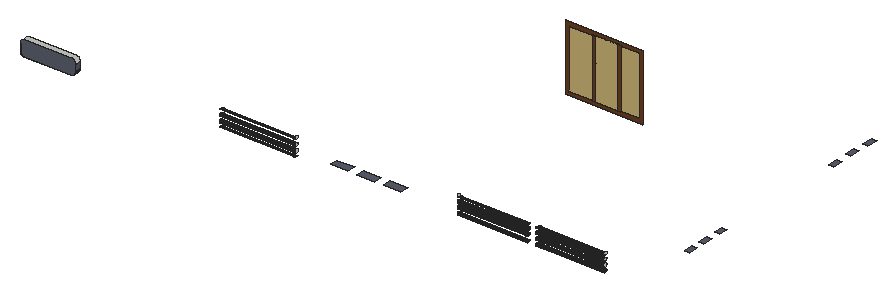
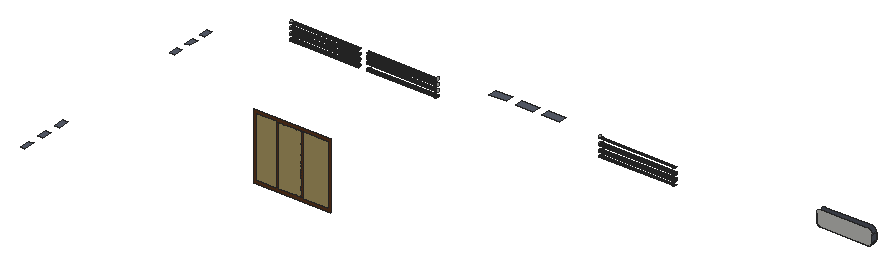
# SketchUp Ruby script. Lengths in inches.
U = 1.inch
M = Sketchup.active_model
def pt(a) = Geom::Point3d.new(a.map { |v| v * U })
def face(e, loops, mat)
  f = e.add_face(loops[0].map { |a| pt(a) })
  loops[1..].each { |l| e.add_face(l.map { |a| pt(a) }).erase! }
  f.material = f.back_material = mat if mat
  f
end
# faces: each face lists its corners as indices into pts; further lists are holes
def faces(e, pts, list, mat = nil) = list.each { |f| face(e, (f[0].is_a?(Array) ? f : [f]).map { |l| l.map { |i| pts[i] } }, mat) }
# xy, xz, yz: faces in a plane at the given z, y or x. An outline is a flat list of corners, or four numbers for a rectangle; further outlines are holes
def ring(l) = l.size == 4 ? [[l[0], l[1]], [l[2], l[1]], [l[2], l[3]], [l[0], l[3]]] : l.each_slice(2).to_a
def flat(e, list, mat, &to3) = list.each { |f| face(e, (f[0].is_a?(Array) ? f : [f]).map { |l| ring(l).map { |u, v| to3.(u, v) } }, mat) }
def xy(e, z, list, mat = nil) = flat(e, list, mat) { |x, y| [x, y, z] }
def xz(e, y, list, mat = nil) = flat(e, list, mat) { |x, z| [x, y, z] }
def yz(e, x, list, mat = nil) = flat(e, list, mat) { |y, z| [x, y, z] }
def lines(e, pts, list) = list.each { |a, b| e.add_line(pt(pts[a]), pt(pts[b])) }
# prism: a flat outline (further loops are holes) pulled along v
def prism(e, loops, v, mat = nil)
  f = face(e, loops, mat); d = Geom::Vector3d.new(v.map { |x| x * U })
  f.pushpull(f.normal.samedirection?(d) ? d.length : -d.length)
end
def box(e, o, s, mat = nil) = prism(e, [[o, [o[0] + s[0], o[1], o[2]], [o[0] + s[0], o[1] + s[1], o[2]], [o[0], o[1] + s[1], o[2]]]], [0, 0, s[2]], mat)
def at(x, y, z, deg = 0) = Geom::Transformation.translation(pt([x, y, z])) * Geom::Transformation.rotation(ORIGIN, Z_AXIS, deg.degrees)
def axes(o, x, y, z) = Geom::Transformation.new([*x, 0, *y, 0, *z, 0, *pt(o).to_a, 1])
def part(name) = M.definitions.add(name)
# library, detail: a bought-in or finely detailed component or shape, given as its bounding box
def library(name, o, s) = part(name).tap { |d| box(d.entities, o, s) }
def detail(e, o, s) = box(e.add_group.entities, o, s)
def put(e, d, t, mat = nil) = e.add_instance(d, t).tap { |i| i.material = mat if mat }
def group(e, t, mat = nil) = e.add_group.tap { |g| g.transformation = t; g.material = mat if mat }.entities
root = M.entities
M.materials.add("[Color M07]").color = [58, 58, 58]
M.materials.add("[Formica Laminate Dark]").color = [89, 94, 107]
M.materials.add("[Window Covering 02]").color = [199, 178, 115]
M.materials.add("[Wood Veneer 01]").color = [107, 62, 33]
xy(root,135.12,[[23.08,274.68,149.38,289.93]],"[Formica Laminate Dark]")
xy(root,149.91,[[1639.03,943.34,1652.28,971.59],[1639.03,1000.59,1652.28,1028.84],[1639.03,1058.41,1652.28,1086.66]],"[Formica Laminate Dark]")
xy(root,155.0625,[[1639.03,462.79,1652.28,487.66],[1639.03,510.85,1652.28,535.72],[1639.03,562.72,1652.28,587.6]],"[Formica Laminate Dark]")
xy(root,155.26,[[832.8125,288.14,879.5,309.57],[902.5,288.14,949.1875,309.57],[974.4375,288.14,1021.125,309.57]],"[Formica Laminate Dark]")
xz(root,274.68,[[23.08,135.12,149.38,135.12,150.95,135.23,152.5,135.53,153.99,136.04,155.4,136.74,156.71,137.61,157.9,138.65,158.9375,139.84,159.8125,141.15,160.51,142.56,161.02,144.05,161.32,145.6,161.43,147.17,161.43,162.99,161.32,164.68,160.99,166.34,160.44,167.94,159.69,169.46,158.75,170.87,157.64,172.14,156.36,173.26,154.96,174.2,153.4375,174.95,151.83,175.49,150.17,175.82,148.48,175.94,26.4,175.94,24.71,175.82,23.04,175.49,21.4375,174.95,19.91,174.2,18.5,173.25,17.23,172.14,16.11,170.86,15.17,169.45,14.42,167.93,13.87,166.32,13.54,164.66,13.43,162.96,13.43,144.77,13.51,143.51,13.76,142.27,14.16,141.08,14.72,139.95,15.42,138.9,16.25,137.95,17.2,137.12,18.25,136.42,19.38,135.86,20.58,135.45,21.82,135.21]],"[Formica Laminate Dark]")
xz(root,289.93,[[23.08,135.12,21.82,135.21,20.58,135.45,19.38,135.86,18.25,136.42,17.2,137.12,16.25,137.95,15.42,138.9,14.72,139.95,14.16,141.08,13.76,142.27,13.51,143.51,13.43,144.77,13.43,162.96,13.54,164.66,13.87,166.32,14.42,167.93,15.17,169.45,16.11,170.86,17.23,172.14,18.5,173.25,19.91,174.2,21.4375,174.95,23.04,175.49,24.71,175.82,26.4,175.94,148.48,175.94,150.17,175.82,151.83,175.49,153.4375,174.95,154.96,174.2,156.36,173.26,157.64,172.14,158.75,170.87,159.69,169.46,160.44,167.94,160.99,166.34,161.32,164.68,161.43,162.99,161.43,147.17,161.32,145.6,161.02,144.05,160.51,142.56,159.8125,141.15,158.9375,139.84,157.9,138.65,156.71,137.61,155.4,136.74,153.99,136.04,152.5,135.53,150.95,135.23,149.38,135.12]])
xz(root,868.79,[[1005.76,135.02,1068.89,293.73],[1077.3,135.02,1134.57,293.73],[1142.99,135.02,1193.04,293.73]],"[Window Covering 02]")
xz(root,868.79,[[[996.55,125.8125,1202.24,302.9375],[1005.76,135.02,1193.04,293.73]],[1068.89,135.02,1077.3,293.73],[1134.57,135.02,1142.99,293.73]],"[Wood Veneer 01]")
yz(root,13.43,[[274.68,144.77,289.93,162.96]],"[Formica Laminate Dark]")
yz(root,161.43,[[274.68,147.17,289.93,162.99]],"[Formica Laminate Dark]")
yz(root,716.4,[[319.3,129.24,320.31,129.37,321.24,129.76,322.04,130.375,322.66,131.18,323.05,132.11,323.18,133.11,323.05,134.12,322.66,135.05,322.04,135.85,321.24,136.47,320.31,136.86,319.3,136.99,318.3,136.86,317.37,136.47,316.56,135.85,315.95,135.05,315.5625,134.12,315.43,133.11,315.5625,132.11,315.95,131.18,316.56,130.375,317.37,129.76,318.3,129.37],[319.3,144.8,320.31,144.93,321.24,145.32,322.04,145.9375,322.66,146.74,323.05,147.67,323.18,148.68,323.05,149.68,322.66,150.61,322.04,151.42,321.24,152.03,320.31,152.42,319.3,152.55,318.3,152.42,317.37,152.03,316.56,151.42,315.95,150.61,315.5625,149.68,315.43,148.68,315.5625,147.67,315.95,146.74,316.56,145.9375,317.37,145.32,318.3,144.93],[319.3,161.86,320.31,162,321.24,162.38,322.04,163,322.66,163.8,323.05,164.74,323.18,165.74,323.05,166.74,322.66,167.68,322.04,168.48,321.24,169.09,320.31,169.48,319.3,169.61,318.3,169.48,317.37,169.09,316.56,168.48,315.95,167.68,315.5625,166.74,315.43,165.74,315.5625,164.74,315.95,163.8,316.56,163,317.37,162.38,318.3,162]])
yz(root,1134.85,[[337.34,134.02,336.35,134.15,335.43,134.53,334.65,135.13,334.04,135.92,333.66,136.84,333.53,137.83,333.66,138.82,334.04,139.74,334.65,140.53,335.43,141.13,336.35,141.51,337.34,141.64,338.33,141.51,339.25,141.13,340.04,140.53,340.64,139.74,341.02,138.82,341.15,137.83,341.02,136.84,340.64,135.92,340.04,135.13,339.25,134.53,338.33,134.15],[337.34,147.52,336.35,147.65,335.43,148.03,334.65,148.63,334.04,149.42,333.66,150.34,333.53,151.33,333.66,152.32,334.04,153.24,334.65,154.03,335.43,154.63,336.35,155.01,337.34,155.14,338.33,155.01,339.25,154.63,340.04,154.03,340.64,153.24,341.02,152.32,341.15,151.33,341.02,150.34,340.64,149.42,340.04,148.63,339.25,148.03,338.33,147.65],[337.34,161.02,336.35,161.15,335.43,161.53,334.65,162.13,334.04,162.92,333.66,163.84,333.53,164.83,333.66,165.82,334.04,166.74,334.65,167.53,335.43,168.13,336.35,168.51,337.34,168.64,338.33,168.51,339.25,168.13,340.04,167.53,340.64,166.74,341.02,165.82,341.15,164.83,341.02,163.84,340.64,162.92,340.04,162.13,339.25,161.53,338.33,161.15]])
yz(root,1527,[[337.76,132.85,338.75,132.98,339.67,133.36,340.46,133.97,341.0625,134.76,341.44,135.67,341.57,136.66,341.44,137.65,341.0625,138.57,340.46,139.36,339.67,139.96,338.75,140.34,337.76,140.47,336.77,140.34,335.85,139.96,335.06,139.36,334.46,138.57,334.08,137.65,333.95,136.66,334.08,135.67,334.46,134.76,335.06,133.97,335.85,133.36,336.77,132.98],[337.76,146.47,338.75,146.6,339.67,146.98,340.46,147.59,341.0625,148.38,341.44,149.3,341.57,150.29,341.44,151.27,341.0625,152.19,340.46,152.98,339.67,153.59,338.75,153.97,337.76,154.1,336.77,153.97,335.85,153.59,335.06,152.98,334.46,152.19,334.08,151.27,333.95,150.29,334.08,149.3,334.46,148.38,335.06,147.59,335.85,146.98,336.77,146.6],[337.76,160.47,338.75,160.6,339.67,160.98,340.46,161.59,341.0625,162.38,341.44,163.3,341.57,164.29,341.44,165.27,341.0625,166.19,340.46,166.98,339.67,167.59,338.75,167.97,337.76,168.1,336.77,167.97,335.85,167.59,335.06,166.98,334.46,166.19,334.08,165.27,333.95,164.29,334.08,163.3,334.46,162.38,335.06,161.59,335.85,160.98,336.77,160.6]])
p = [[1527,335.06,119.53],[1527,334.46,120.32],[1344.86,334.46,120.32],[1344.86,335.06,119.53],[1527,341.0625,120.32],[1527,340.46,119.53],
  [1344.86,340.46,119.53],[1344.86,341.0625,120.32],[716.4,315.95,119.61],[716.4,316.56,120.42],[513.6,316.56,120.42],[513.6,315.95,119.61],
  [716.4,322.04,120.42],[716.4,322.66,119.61],[513.6,322.66,119.61],[513.6,322.04,120.42],[1134.85,333.66,120.72],[1134.85,334.04,119.8],
  [1322.28,334.04,119.8],[1322.28,333.66,120.72],[1134.85,340.64,119.8],[1134.85,341.02,120.72],[1322.28,341.02,120.72],[1322.28,340.64,119.8],
  [1527,334.08,121.24],[1344.86,334.08,121.24],[1527,341.44,121.24],[1344.86,341.44,121.24],[716.4,317.37,121.03],[513.6,317.37,121.03],
  [716.4,321.24,121.03],[513.6,321.24,121.03],[1134.85,333.53,121.71],[1322.28,333.53,121.71],[1134.85,341.15,121.71],[1322.28,341.15,121.71],
  [716.4,318.3,121.42],[513.6,318.3,121.42],[716.4,320.31,121.42],[513.6,320.31,121.42],[1527,333.95,122.22],[1344.86,333.95,122.22],
  [1527,341.57,122.22],[1344.86,341.57,122.22],[716.4,319.3,121.55],[513.6,319.3,121.55],[1134.85,333.66,122.69],[1322.28,333.66,122.69],
  [1134.85,341.02,122.69],[1322.28,341.02,122.69],[1527,334.08,123.21],[1344.86,334.08,123.21],[1527,341.44,123.21],[1344.86,341.44,123.21],
  [1134.85,334.04,123.61],[1322.28,334.04,123.61],[1134.85,340.64,123.61],[1322.28,340.64,123.61],[1527,334.46,124.13],[1344.86,334.46,124.13],
  [1527,341.0625,124.13],[1344.86,341.0625,124.13],[1134.85,334.65,124.4],[1322.28,334.65,124.4],[1134.85,340.04,124.4],[1322.28,340.04,124.4],
  [1527,335.06,124.92],[1344.86,335.06,124.92],[1527,340.46,124.92],[1344.86,340.46,124.92],[1134.85,335.43,125.01],[1322.28,335.43,125.01],
  [1134.85,339.25,125.01],[1322.28,339.25,125.01],[1527,335.85,125.53],[1344.86,335.85,125.53],[1527,339.67,125.53],[1344.86,339.67,125.53],
  [1134.85,336.35,125.39],[1322.28,336.35,125.39],[1134.85,338.33,125.39],[1322.28,338.33,125.39],[1134.85,337.34,125.52],[1322.28,337.34,125.52],
  [1527,336.77,125.91],[1344.86,336.77,125.91],[1527,338.75,125.91],[1344.86,338.75,125.91],[1527,337.76,126.04],[1344.86,337.76,126.04],
  [716.4,319.3,129.24],[716.4,318.3,129.37],[513.6,318.3,129.37],[513.6,319.3,129.24],[716.4,320.31,129.37],[513.6,320.31,129.37],
  [716.4,317.37,129.76],[513.6,317.37,129.76],[716.4,321.24,129.76],[513.6,321.24,129.76],[716.4,316.56,130.375],[513.6,316.56,130.375],
  [716.4,322.04,130.375],[513.6,322.04,130.375],[716.4,315.95,131.18],[513.6,315.95,131.18],[716.4,322.66,131.18],[513.6,322.66,131.18],
  [716.4,315.5625,132.11],[513.6,315.5625,132.11],[716.4,323.05,132.11],[513.6,323.05,132.11],[716.4,315.43,133.11],[513.6,315.43,133.11],
  [716.4,323.18,133.11],[513.6,323.18,133.11],[1527,337.76,132.85],[1527,336.77,132.98],[1344.86,336.77,132.98],[1344.86,337.76,132.85],
  [1527,338.75,132.98],[1344.86,338.75,132.98],[1527,335.85,133.36],[1344.86,335.85,133.36],[1527,339.67,133.36],[1344.86,339.67,133.36],
  [716.4,315.5625,134.12],[513.6,315.5625,134.12],[716.4,323.05,134.12],[513.6,323.05,134.12],[1527,335.06,133.97],[1344.86,335.06,133.97],
  [1527,340.46,133.97],[1344.86,340.46,133.97],[1527,334.46,134.76],[1344.86,334.46,134.76],[1134.85,336.35,134.15],[1134.85,337.34,134.02],
  [1322.28,337.34,134.02],[1322.28,336.35,134.15],[1134.85,338.33,134.15],[1322.28,338.33,134.15],[1527,341.0625,134.76],[1344.86,341.0625,134.76],
  [716.4,315.95,135.05],[513.6,315.95,135.05],[716.4,322.66,135.05],[513.6,322.66,135.05],[1134.85,335.43,134.53],[1322.28,335.43,134.53],
  [1134.85,339.25,134.53],[1322.28,339.25,134.53],[1134.85,334.65,135.13],[1322.28,334.65,135.13],[1134.85,340.04,135.13],[1322.28,340.04,135.13],
  [1527,334.08,135.67],[1344.86,334.08,135.67],[1527,341.44,135.67],[1344.86,341.44,135.67],[21.82,289.93,135.21],[23.08,289.93,135.12],
  [23.08,274.68,135.12],[21.82,274.68,135.21],[149.38,289.93,135.12],[150.95,289.93,135.23],[150.95,274.68,135.23],[149.38,274.68,135.12],
  [716.4,316.56,135.85],[513.6,316.56,135.85],[716.4,322.04,135.85],[513.6,322.04,135.85],[1134.85,334.04,135.92],[1322.28,334.04,135.92],
  [1134.85,340.64,135.92],[1322.28,340.64,135.92],[20.58,289.93,135.45],[20.58,274.68,135.45],[152.5,289.93,135.53],[152.5,274.68,135.53],
  [19.38,289.93,135.86],[19.38,274.68,135.86],[153.99,289.93,136.04],[153.99,274.68,136.04],[1527,333.95,136.66],[1344.86,333.95,136.66],
  [1527,341.57,136.66],[1344.86,341.57,136.66],[18.25,289.93,136.42],[18.25,274.68,136.42],[716.4,317.37,136.47],[513.6,317.37,136.47],
  [716.4,321.24,136.47],[513.6,321.24,136.47],[1134.85,333.66,136.84],[1322.28,333.66,136.84],[1134.85,341.02,136.84],[1322.28,341.02,136.84],
  [155.4,289.93,136.74],[155.4,274.68,136.74],[17.2,289.93,137.12],[17.2,274.68,137.12],[716.4,318.3,136.86],[513.6,318.3,136.86],
  [716.4,320.31,136.86],[513.6,320.31,136.86],[156.71,289.93,137.61],[156.71,274.68,137.61],[1527,334.08,137.65],[1344.86,334.08,137.65],
  [1527,341.44,137.65],[1344.86,341.44,137.65],[1134.85,333.53,137.83],[1322.28,333.53,137.83],[1134.85,341.15,137.83],[1322.28,341.15,137.83],
  [716.4,319.3,136.99],[513.6,319.3,136.99],[16.25,289.93,137.95],[16.25,274.68,137.95],[157.9,289.93,138.65],[157.9,274.68,138.65],
  [1527,334.46,138.57],[1344.86,334.46,138.57],[1527,341.0625,138.57],[1344.86,341.0625,138.57],[1134.85,333.66,138.82],[1322.28,333.66,138.82],
  [1134.85,341.02,138.82],[1322.28,341.02,138.82],[15.42,289.93,138.9],[15.42,274.68,138.9],[1527,335.06,139.36],[1344.86,335.06,139.36],
  [1527,340.46,139.36],[1344.86,340.46,139.36],[158.9375,289.93,139.84],[158.9375,274.68,139.84],[1134.85,334.04,139.74],[1322.28,334.04,139.74],
  [1134.85,340.64,139.74],[1322.28,340.64,139.74],[14.72,289.93,139.95],[14.72,274.68,139.95],[1527,335.85,139.96],[1344.86,335.85,139.96],
  [1527,339.67,139.96],[1344.86,339.67,139.96],[1134.85,334.65,140.53],[1322.28,334.65,140.53],[1134.85,340.04,140.53],[1322.28,340.04,140.53],
  [159.8125,289.93,141.15],[159.8125,274.68,141.15],[14.16,289.93,141.08],[14.16,274.68,141.08],[1527,336.77,140.34],[1344.86,336.77,140.34],
  [1527,338.75,140.34],[1344.86,338.75,140.34],[1527,337.76,140.47],[1344.86,337.76,140.47],[1134.85,335.43,141.13],[1322.28,335.43,141.13],
  [1134.85,339.25,141.13],[1322.28,339.25,141.13],[13.76,289.93,142.27],[13.76,274.68,142.27],[160.51,289.93,142.56],[160.51,274.68,142.56],
  [1134.85,336.35,141.51],[1322.28,336.35,141.51],[1134.85,338.33,141.51],[1322.28,338.33,141.51],[1134.85,337.34,141.64],[1322.28,337.34,141.64],
  [13.51,289.93,143.51],[13.51,274.68,143.51],[161.02,289.93,144.05],[161.02,274.68,144.05],[13.43,289.93,144.77],[13.43,274.68,144.77],
  [161.32,289.93,145.6],[161.32,274.68,145.6],[716.4,319.3,144.8],[716.4,318.3,144.93],[513.6,318.3,144.93],[513.6,319.3,144.8],
  [716.4,320.31,144.93],[513.6,320.31,144.93],[716.4,317.37,145.32],[513.6,317.37,145.32],[716.4,321.24,145.32],[513.6,321.24,145.32],
  [716.4,316.56,145.9375],[513.6,316.56,145.9375],[716.4,322.04,145.9375],[513.6,322.04,145.9375],[161.43,289.93,147.17],[161.43,274.68,147.17],
  [716.4,315.95,146.74],[513.6,315.95,146.74],[716.4,322.66,146.74],[513.6,322.66,146.74],[1527,337.76,146.47],[1527,336.77,146.6],
  [1344.86,336.77,146.6],[1344.86,337.76,146.47],[1527,338.75,146.6],[1344.86,338.75,146.6],[1527,335.85,146.98],[1344.86,335.85,146.98],
  [1527,339.67,146.98],[1344.86,339.67,146.98],[716.4,315.5625,147.67],[513.6,315.5625,147.67],[716.4,323.05,147.67],[513.6,323.05,147.67],
  [1527,335.06,147.59],[1344.86,335.06,147.59],[1527,340.46,147.59],[1344.86,340.46,147.59],[1134.85,336.35,147.65],[1134.85,337.34,147.52],
  [1322.28,337.34,147.52],[1322.28,336.35,147.65],[1134.85,338.33,147.65],[1322.28,338.33,147.65],[1527,334.46,148.38],[1344.86,334.46,148.38],
  [1134.85,335.43,148.03],[1322.28,335.43,148.03],[1134.85,339.25,148.03],[1322.28,339.25,148.03],[1527,341.0625,148.38],[1344.86,341.0625,148.38],
  [716.4,315.43,148.68],[513.6,315.43,148.68],[716.4,323.18,148.68],[513.6,323.18,148.68],[1134.85,334.65,148.63],[1322.28,334.65,148.63],
  [1134.85,340.04,148.63],[1322.28,340.04,148.63],[1527,334.08,149.3],[1344.86,334.08,149.3],[1527,341.44,149.3],[1344.86,341.44,149.3],
  [1134.85,334.04,149.42],[1322.28,334.04,149.42],[1134.85,340.64,149.42],[1322.28,340.64,149.42],[716.4,315.5625,149.68],[513.6,315.5625,149.68],
  [716.4,323.05,149.68],[513.6,323.05,149.68],[1527,333.95,150.29],[1344.86,333.95,150.29],[1527,341.57,150.29],[1344.86,341.57,150.29],
  [1134.85,333.66,150.34],[1322.28,333.66,150.34],[1134.85,341.02,150.34],[1322.28,341.02,150.34],[716.4,315.95,150.61],[513.6,315.95,150.61],
  [716.4,322.66,150.61],[513.6,322.66,150.61],[1134.85,333.53,151.33],[1322.28,333.53,151.33],[1527,334.08,151.27],[1344.86,334.08,151.27],
  [1134.85,341.15,151.33],[1322.28,341.15,151.33],[1527,341.44,151.27],[1344.86,341.44,151.27],[716.4,316.56,151.42],[513.6,316.56,151.42],
  [716.4,322.04,151.42],[513.6,322.04,151.42],[1134.85,333.66,152.32],[1322.28,333.66,152.32],[1527,334.46,152.19],[1344.86,334.46,152.19],
  [1134.85,341.02,152.32],[1322.28,341.02,152.32],[1527,341.0625,152.19],[1344.86,341.0625,152.19],[716.4,317.37,152.03],[513.6,317.37,152.03],
  [716.4,321.24,152.03],[513.6,321.24,152.03],[716.4,318.3,152.42],[513.6,318.3,152.42],[716.4,320.31,152.42],[513.6,320.31,152.42],
  [1527,335.06,152.98],[1344.86,335.06,152.98],[1527,340.46,152.98],[1344.86,340.46,152.98],[1134.85,334.04,153.24],[1322.28,334.04,153.24],
  [1134.85,340.64,153.24],[1322.28,340.64,153.24],[716.4,319.3,152.55],[513.6,319.3,152.55],[1527,335.85,153.59],[1344.86,335.85,153.59],
  [1527,339.67,153.59],[1344.86,339.67,153.59],[1134.85,334.65,154.03],[1322.28,334.65,154.03],[1134.85,340.04,154.03],[1322.28,340.04,154.03],
  [1527,336.77,153.97],[1344.86,336.77,153.97],[1527,338.75,153.97],[1344.86,338.75,153.97],[1134.85,335.43,154.63],[1322.28,335.43,154.63],
  [1527,337.76,154.1],[1344.86,337.76,154.1],[1134.85,339.25,154.63],[1322.28,339.25,154.63],[1134.85,336.35,155.01],[1322.28,336.35,155.01],
  [1134.85,338.33,155.01],[1322.28,338.33,155.01],[1134.85,337.34,155.14],[1322.28,337.34,155.14],[1527,337.76,160.47],[1527,336.77,160.6],
  [1344.86,336.77,160.6],[1344.86,337.76,160.47],[1527,338.75,160.6],[1344.86,338.75,160.6],[1527,335.85,160.98],[1344.86,335.85,160.98],
  [1527,339.67,160.98],[1344.86,339.67,160.98],[1527,335.06,161.59],[1344.86,335.06,161.59],[1134.85,336.35,161.15],[1134.85,337.34,161.02],
  [1322.28,337.34,161.02],[1322.28,336.35,161.15],[1134.85,338.33,161.15],[1322.28,338.33,161.15],[1527,340.46,161.59],[1344.86,340.46,161.59],
  [1134.85,335.43,161.53],[1322.28,335.43,161.53],[1134.85,339.25,161.53],[1322.28,339.25,161.53],[1134.85,334.65,162.13],[1322.28,334.65,162.13],
  [1134.85,340.04,162.13],[1322.28,340.04,162.13],[1527,334.46,162.38],[1344.86,334.46,162.38],[1527,341.0625,162.38],[1344.86,341.0625,162.38],
  [716.4,319.3,161.86],[716.4,318.3,162],[513.6,318.3,162],[513.6,319.3,161.86],[716.4,320.31,162],[513.6,320.31,162],
  [716.4,317.37,162.38],[513.6,317.37,162.38],[716.4,321.24,162.38],[513.6,321.24,162.38],[1134.85,334.04,162.92],[1322.28,334.04,162.92],
  [1134.85,340.64,162.92],[1322.28,340.64,162.92],[716.4,316.56,163],[513.6,316.56,163],[716.4,322.04,163],[513.6,322.04,163],
  [1527,334.08,163.3],[1344.86,334.08,163.3],[1527,341.44,163.3],[1344.86,341.44,163.3],[1134.85,333.66,163.84],[1322.28,333.66,163.84],
  [1134.85,341.02,163.84],[1322.28,341.02,163.84],[13.54,289.93,164.66],[13.43,289.93,162.96],[13.43,274.68,162.96],[13.54,274.68,164.66],
  [161.43,289.93,162.99],[161.32,289.93,164.68],[161.32,274.68,164.68],[161.43,274.68,162.99],[716.4,315.95,163.8],[513.6,315.95,163.8],
  [716.4,322.66,163.8],[513.6,322.66,163.8],[1527,333.95,164.29],[1344.86,333.95,164.29],[1527,341.57,164.29],[1344.86,341.57,164.29]]
faces(root,p,[[0,1,2,3],[4,5,6,7],[8,9,10,11],[12,13,14,15],[16,17,18,19],[20,21,22,23],[1,24,25,2],[26,4,7,27],
  [9,28,29,10],[30,12,15,31],[32,16,19,33],[21,34,35,22],[28,36,37,29],[38,30,31,39],[24,40,41,25],[42,26,27,43],
  [36,44,45,37],[44,38,39,45],[46,32,33,47],[34,48,49,35],[40,50,51,41],[52,42,43,53],[54,46,47,55],[48,56,57,49],
  [50,58,59,51],[60,52,53,61],[62,54,55,63],[56,64,65,57],[58,66,67,59],[68,60,61,69],[70,62,63,71],[64,72,73,65],
  [66,74,75,67],[76,68,69,77],[78,70,71,79],[72,80,81,73],[82,78,79,83],[80,82,83,81],[74,84,85,75],[86,76,77,87],
  [84,88,89,85],[88,86,87,89],[90,91,92,93],[94,90,93,95],[91,96,97,92],[98,94,95,99],[96,100,101,97],[102,98,99,103],
  [100,104,105,101],[106,102,103,107],[104,108,109,105],[110,106,107,111],[108,112,113,109],[114,110,111,115],[116,117,118,119],[120,116,119,121],
  [117,122,123,118],[124,120,121,125],[112,126,127,113],[128,114,115,129],[122,130,131,123],[132,124,125,133],[130,134,135,131],[136,137,138,139],
  [137,140,141,138],[142,132,133,143],[126,144,145,127],[146,128,129,147],[148,136,139,149],[140,150,151,141],[152,148,149,153],[150,154,155,151],
  [134,156,157,135],[158,142,143,159],[144,168,169,145],[170,146,147,171],[172,152,153,173],[154,174,175,155],[156,184,185,157],[186,158,159,187],
  [168,190,191,169],[192,170,171,193],[194,172,173,195],[174,196,197,175],[190,202,203,191],[204,192,193,205],[184,208,209,185],[210,186,187,211],
  [212,194,195,213],[196,214,215,197],[202,216,217,203],[216,204,205,217],[208,222,223,209],[224,210,211,225],[226,212,213,227],[214,228,229,215],
  [222,232,233,223],[234,224,225,235],[238,226,227,239],[228,240,241,229],[232,244,245,233],[246,234,235,247],[248,238,239,249],[240,250,251,241],
  [244,256,257,245],[258,246,247,259],[256,260,261,257],[260,258,259,261],[262,248,249,263],[250,264,265,251],[270,262,263,271],[264,272,273,265],
  [274,270,271,275],[272,274,275,273],[284,285,286,287],[288,284,287,289],[285,290,291,286],[292,288,289,293],[290,294,295,291],[296,292,293,297],
  [294,300,301,295],[302,296,297,303],[304,305,306,307],[308,304,307,309],[305,310,311,306],[312,308,309,313],[300,314,315,301],[316,302,303,317],
  [310,318,319,311],[320,312,313,321],[322,323,324,325],[323,326,327,324],[318,328,329,319],[330,322,325,331],[326,332,333,327],[334,320,321,335],
  [314,336,337,315],[338,316,317,339],[340,330,331,341],[332,342,343,333],[328,344,345,329],[346,334,335,347],[348,340,341,349],[342,350,351,343],
  [336,352,353,337],[354,338,339,355],[344,356,357,345],[358,346,347,359],[360,348,349,361],[350,362,363,351],[352,364,365,353],[366,354,355,367],
  [368,360,361,369],[356,370,371,357],[362,372,373,363],[374,358,359,375],[364,376,377,365],[378,366,367,379],[380,368,369,381],[370,382,383,371],
  [372,384,385,373],[386,374,375,387],[376,388,389,377],[390,378,379,391],[388,392,393,389],[394,390,391,395],[382,396,397,383],[398,386,387,399],
  [400,380,381,401],[384,402,403,385],[392,404,405,393],[404,394,395,405],[396,406,407,397],[408,398,399,409],[410,400,401,411],[402,412,413,403],
  [406,414,415,407],[416,408,409,417],[418,410,411,419],[414,420,421,415],[420,416,417,421],[412,422,423,413],[424,418,419,425],[422,426,427,423],
  [428,424,425,429],[426,428,429,427],[430,431,432,433],[434,430,433,435],[431,436,437,432],[438,434,435,439],[436,440,441,437],[442,443,444,445],
  [443,446,447,444],[448,438,439,449],[450,442,445,451],[446,452,453,447],[454,450,451,455],[452,456,457,453],[440,458,459,441],[460,448,449,461],
  [462,463,464,465],[466,462,465,467],[463,468,469,464],[470,466,467,471],[472,454,455,473],[456,474,475,457],[468,476,477,469],[478,470,471,479],
  [458,480,481,459],[482,460,461,483],[484,472,473,485],[474,486,487,475],[476,496,497,477],[498,478,479,499],[480,500,501,481],[502,482,483,503]],"[Color M07]")
faces(root,p,[[160,161,162,163],[164,165,166,167],[176,160,163,177],[165,178,179,166],[180,176,177,181],[178,182,183,179],[188,180,181,189],[182,198,199,183],
  [200,188,189,201],[198,206,207,199],[218,200,201,219],[206,220,221,207],[230,218,219,231],[220,236,237,221],[242,230,231,243],[236,252,253,237],
  [254,242,243,255],[266,254,255,267],[252,268,269,253],[276,266,267,277],[268,278,279,269],[280,276,277,281],[278,282,283,279],[282,298,299,283],
  [488,489,490,491],[492,493,494,495]],"[Formica Laminate Dark]")
